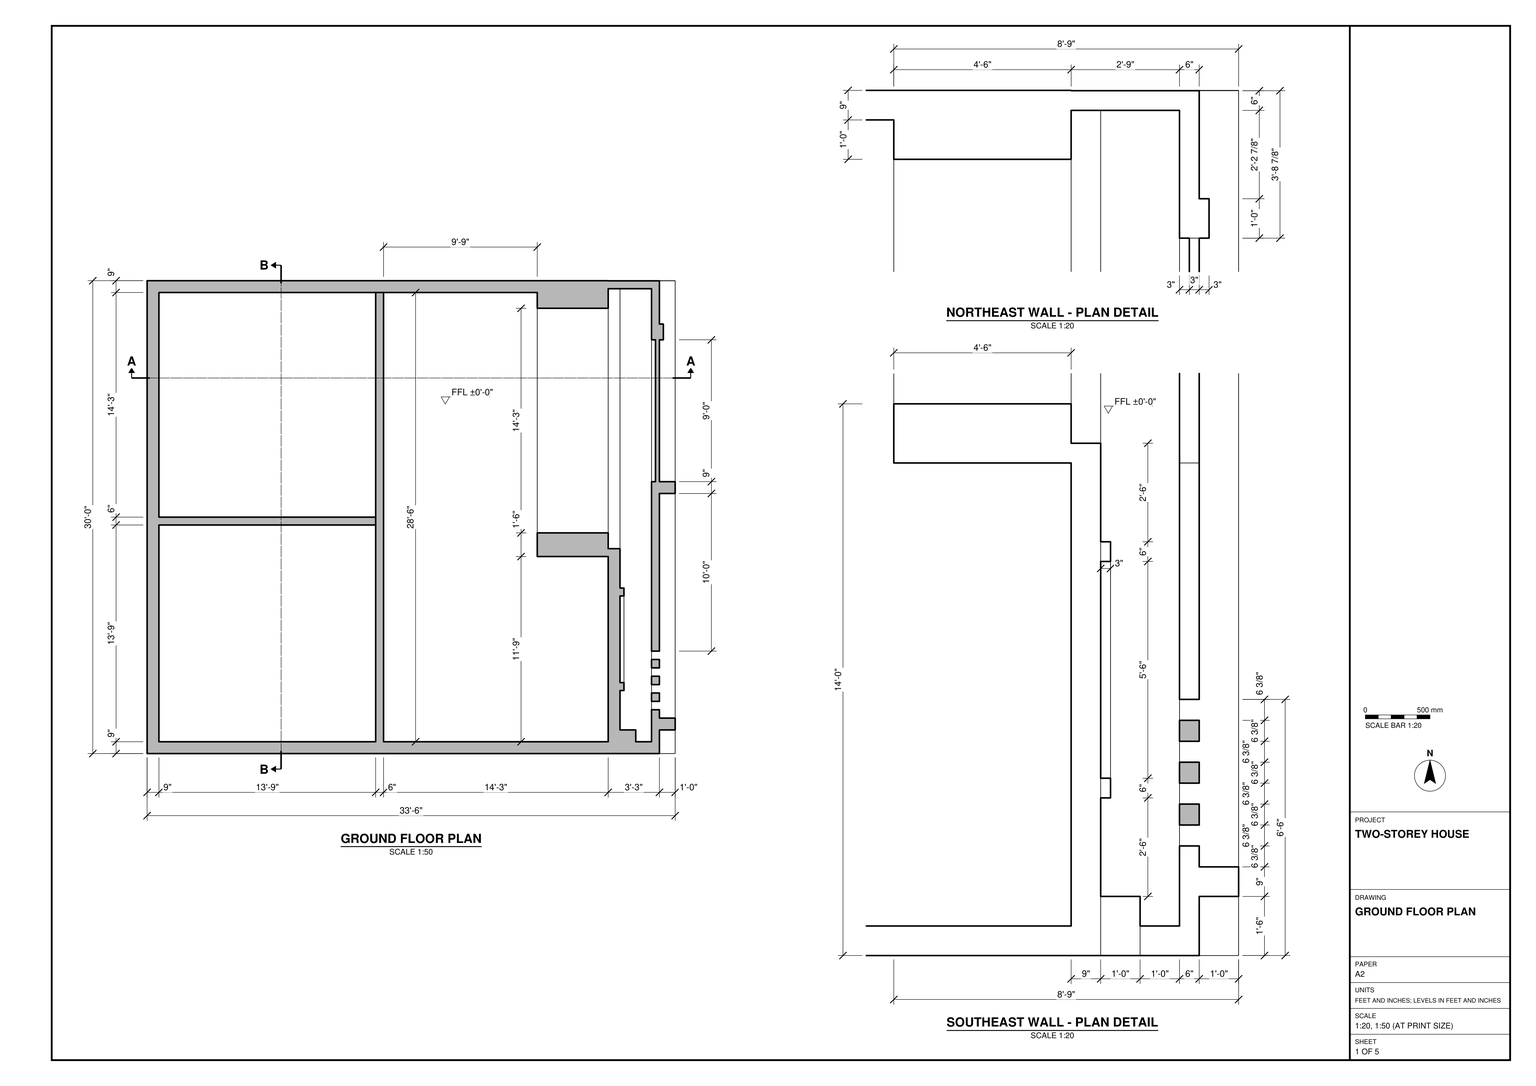
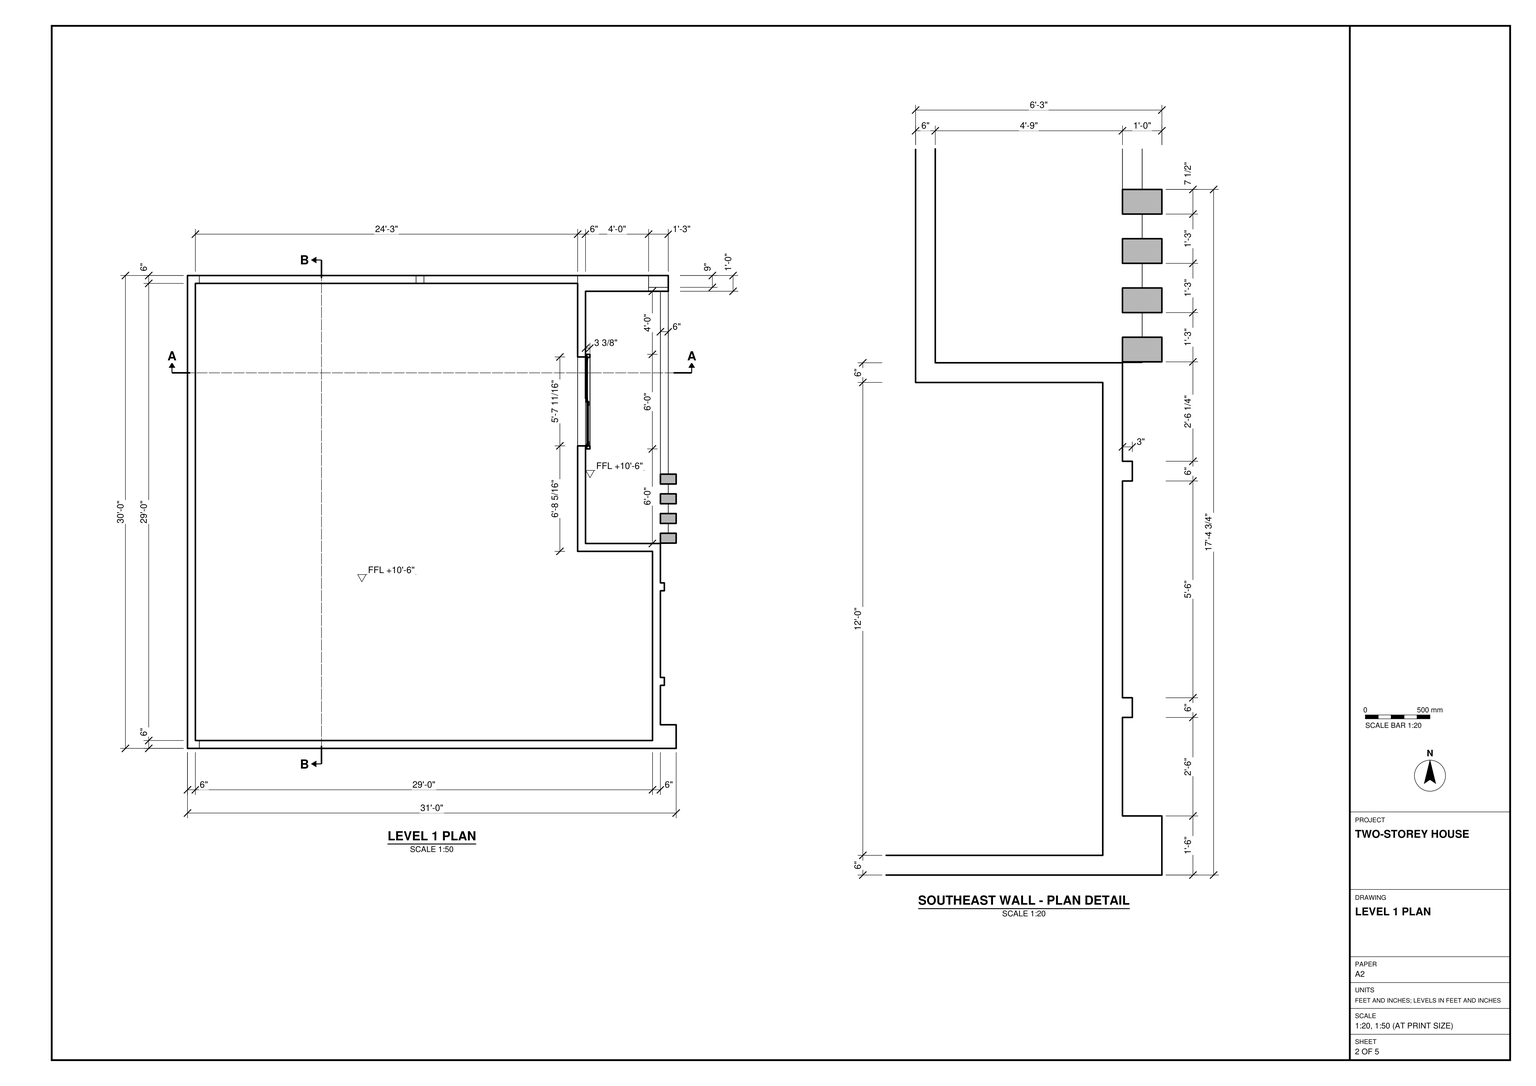
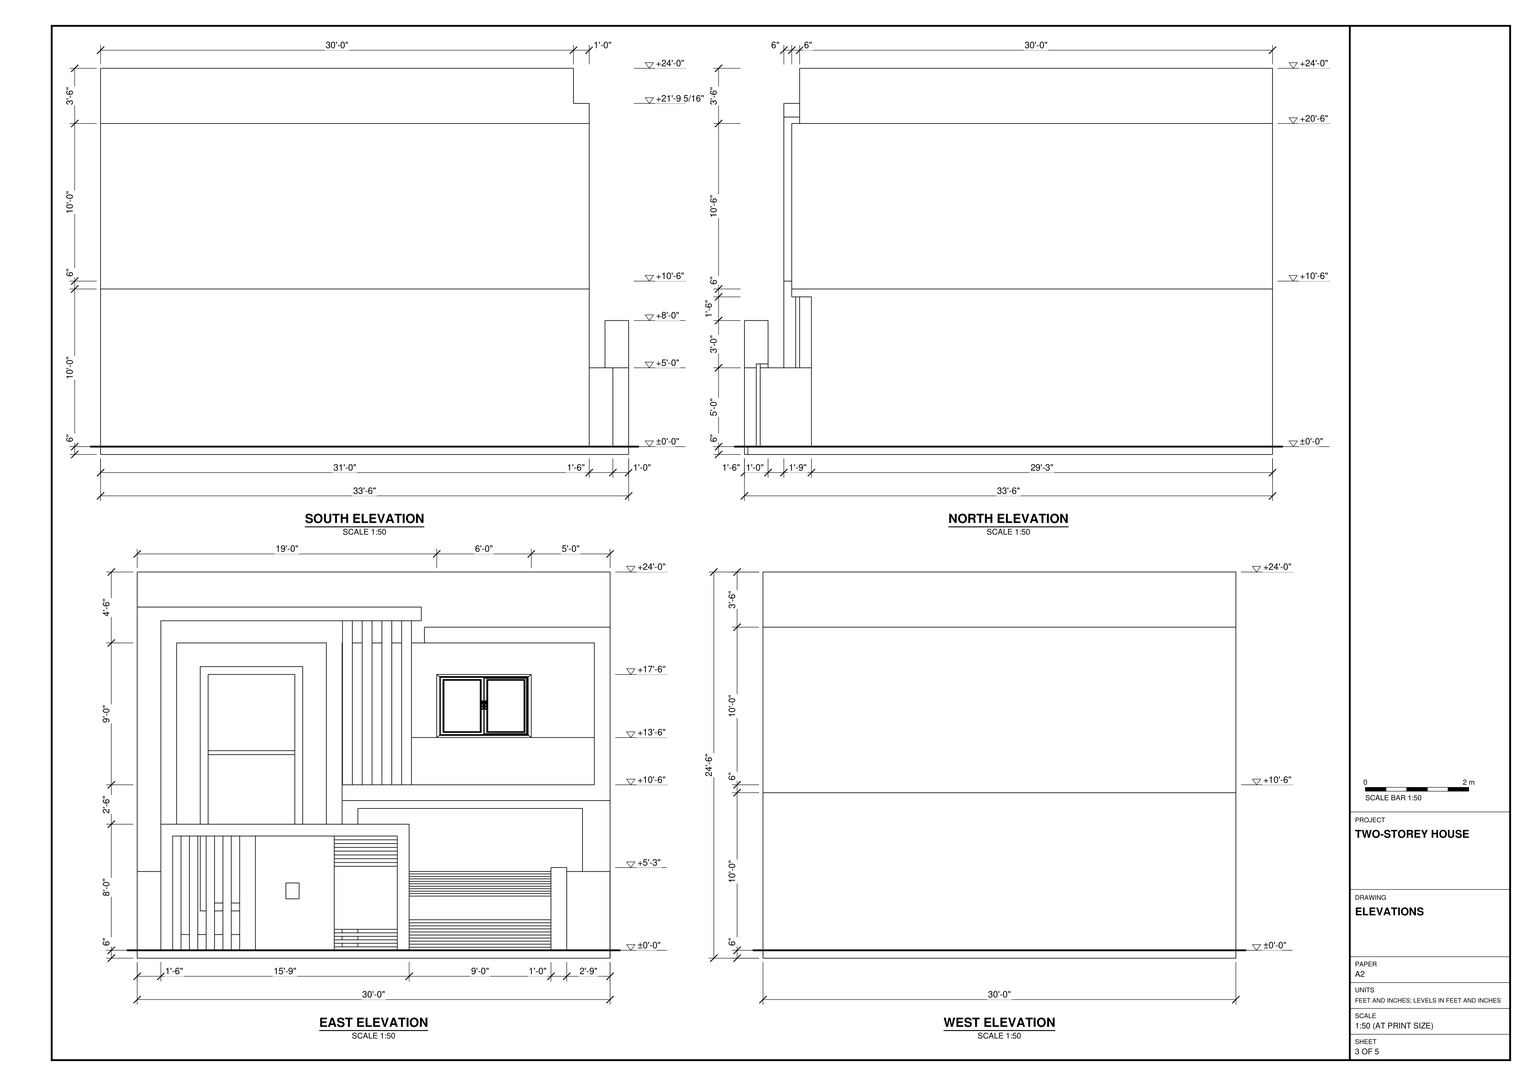
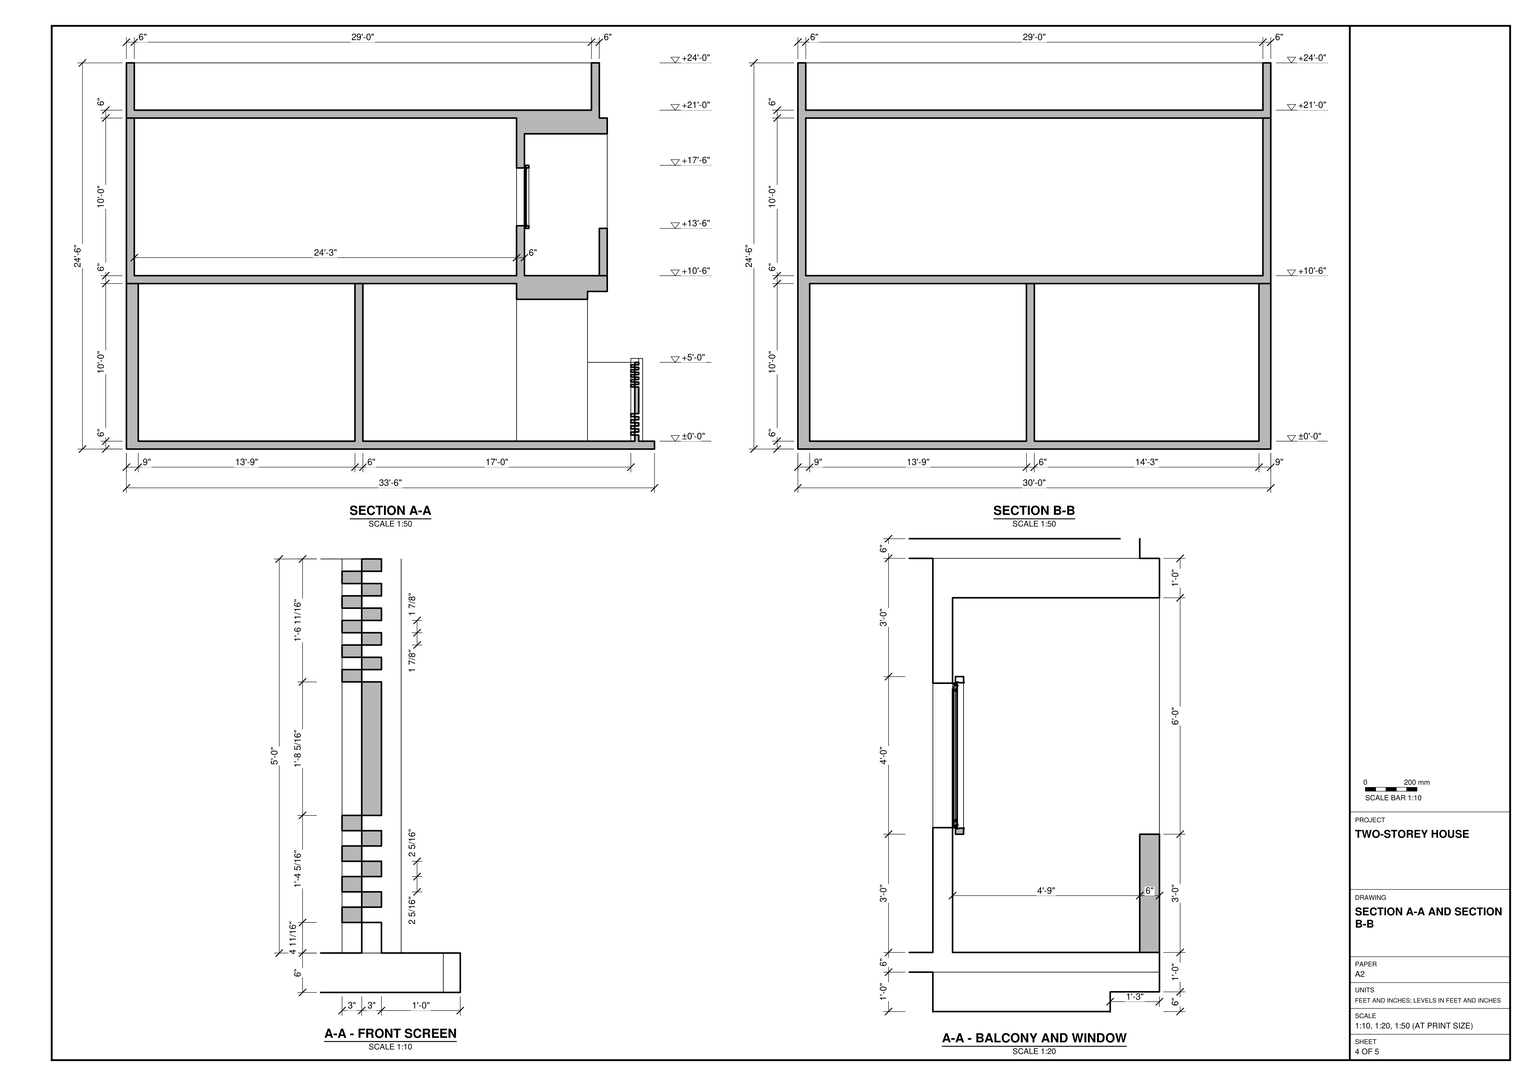
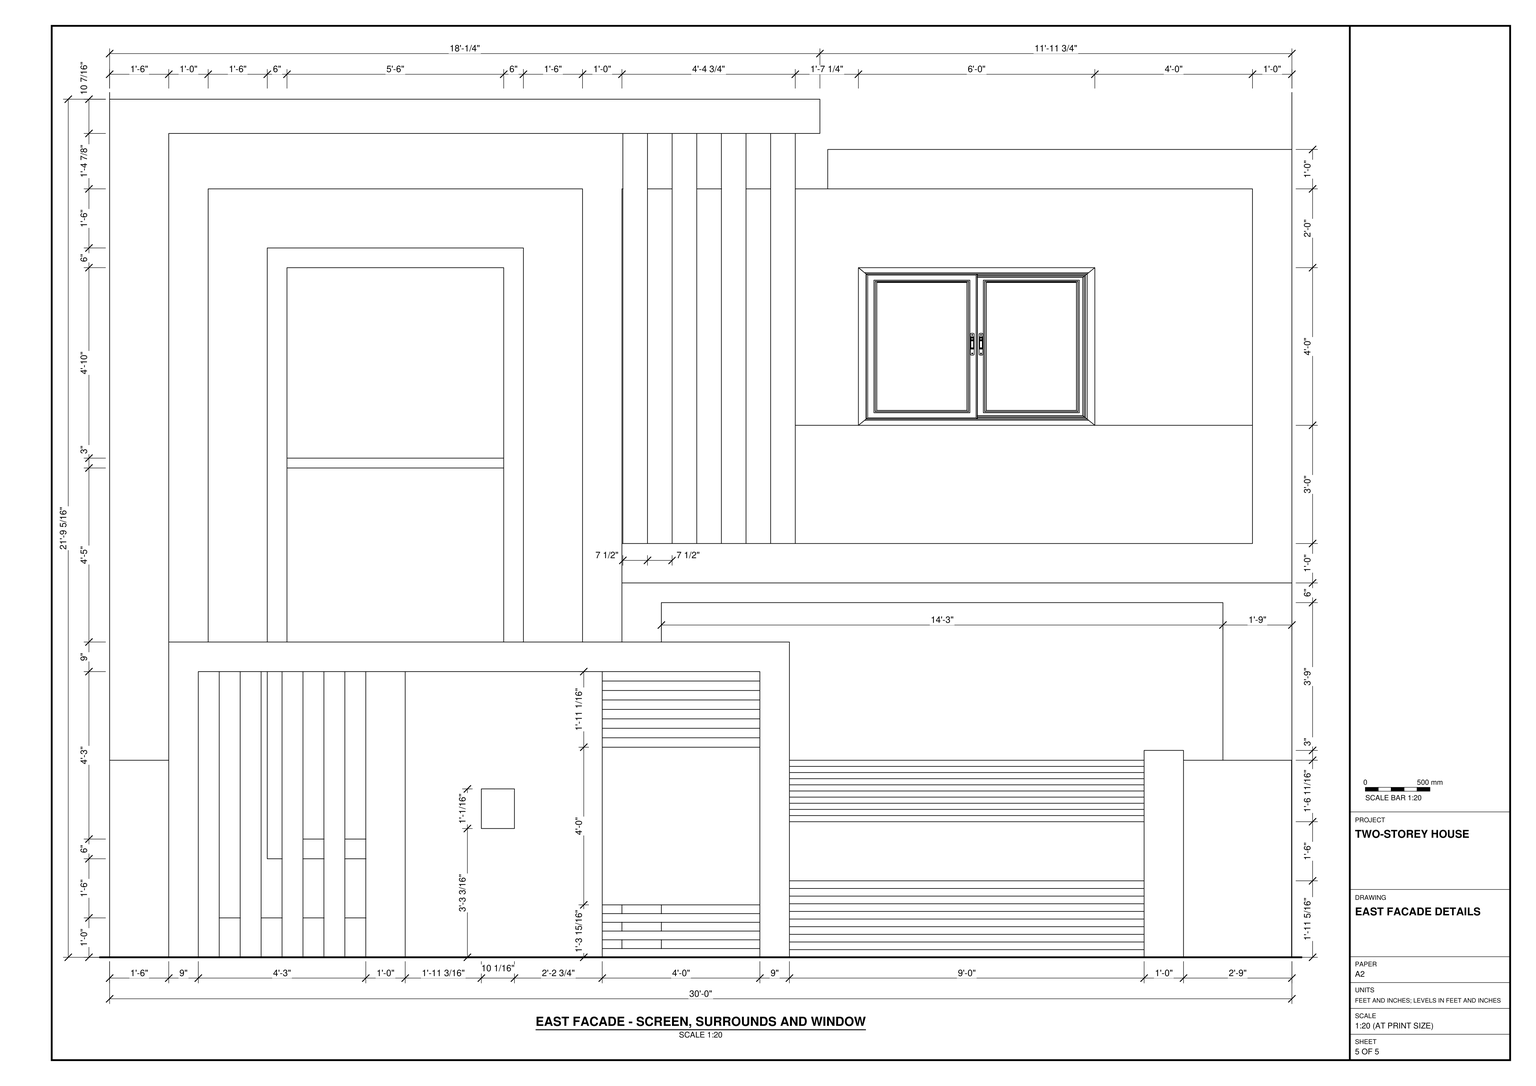
Build the two-storey house in SketchUp from task_files/diagram_01.pdf. Work in feet and inches. Orient the model with east–west along the x-axis and north–south along the y-axis. The overall extents, including the projecting east frontage and the base slab, are 33'-6" by 30'-0" by 24'-6". Set the ground finished floor at ±0'-0" and the upper finished floor at +10'-6". The parapet top is at +24'-0"; the overall height includes the 6" slab below the ground floor datum.

Follow the plans for wall positions and thicknesses. On the ground floor, use the north–south partition and its westward return to define the two western rooms. Use the enlarged east wall details to model the recesses and projections rather than treating the frontage as a single flat wall. Form the upper floor slab, the stepped upper perimeter, the flat roof and its parapet. Match the east elevation’s projecting frames, vertical fins, recessed window and lower frontage screen, keeping the solid panels distinct from the slatted sections.

Keep walls, slabs and roof as separate groups or components. Keep any furniture or joinery shown as separate pieces and use components for repeated parts such as matching fins. Any decor or loose items shown may be represented by suitable library components. Save one SketchUp model as output_files/two_storey_house_with_a_screened_east_facade.skp.

# SketchUp Ruby script. Lengths in inches.
U = 1.inch
M = Sketchup.active_model
def pt(a) = Geom::Point3d.new(a.map { |v| v * U })
def face(e, loops, mat)
  f = e.add_face(loops[0].map { |a| pt(a) })
  loops[1..].each { |l| e.add_face(l.map { |a| pt(a) }).erase! }
  f.material = f.back_material = mat if mat
  f
end
# faces: each face lists its corners as indices into pts; further lists are holes
def faces(e, pts, list, mat = nil) = list.each { |f| face(e, (f[0].is_a?(Array) ? f : [f]).map { |l| l.map { |i| pts[i] } }, mat) }
# xy, xz, yz: faces in a plane at the given z, y or x. An outline is a flat list of corners, or four numbers for a rectangle; further outlines are holes
def ring(l) = l.size == 4 ? [[l[0], l[1]], [l[2], l[1]], [l[2], l[3]], [l[0], l[3]]] : l.each_slice(2).to_a
def flat(e, list, mat, &to3) = list.each { |f| face(e, (f[0].is_a?(Array) ? f : [f]).map { |l| ring(l).map { |u, v| to3.(u, v) } }, mat) }
def xy(e, z, list, mat = nil) = flat(e, list, mat) { |x, y| [x, y, z] }
def xz(e, y, list, mat = nil) = flat(e, list, mat) { |x, z| [x, y, z] }
def yz(e, x, list, mat = nil) = flat(e, list, mat) { |y, z| [x, y, z] }
def lines(e, pts, list) = list.each { |a, b| e.add_line(pt(pts[a]), pt(pts[b])) }
# prism: a flat outline (further loops are holes) pulled along v
def prism(e, loops, v, mat = nil)
  f = face(e, loops, mat); d = Geom::Vector3d.new(v.map { |x| x * U })
  f.pushpull(f.normal.samedirection?(d) ? d.length : -d.length)
end
def box(e, o, s, mat = nil) = prism(e, [[o, [o[0] + s[0], o[1], o[2]], [o[0] + s[0], o[1] + s[1], o[2]], [o[0], o[1] + s[1], o[2]]]], [0, 0, s[2]], mat)
def at(x, y, z, deg = 0) = Geom::Transformation.translation(pt([x, y, z])) * Geom::Transformation.rotation(ORIGIN, Z_AXIS, deg.degrees)
def axes(o, x, y, z) = Geom::Transformation.new([*x, 0, *y, 0, *z, 0, *pt(o).to_a, 1])
def part(name) = M.definitions.add(name)
# library, detail: a bought-in or finely detailed component or shape, given as its bounding box
def library(name, o, s) = part(name).tap { |d| box(d.entities, o, s) }
def detail(e, o, s) = box(e.add_group.entities, o, s)
def put(e, d, t, mat = nil) = e.add_instance(d, t).tap { |i| i.material = mat if mat }
def group(e, t, mat = nil) = e.add_group.tap { |g| g.transformation = t; g.material = mat if mat }.entities
root = M.entities
M.materials.add("Carpet_04_1K").color = [43, 65, 85]
M.materials.add("Glass_Basic_01").color = [161, 173, 186]
M.materials["Glass_Basic_01"].alpha = 0.25
M.materials.add("H01_Misty_Ice").color = [204, 255, 255]
M.materials.add("I01_Sky_Frost").color = [241, 228, 255]
M.materials.add("J07_Grape_Bloom").color = [73, 0, 153]
M.materials.add("M01_Silver_Fog").color = [224, 224, 224]
M.materials.add("Wood_Veneer_15_1K").color = [103, 69, 45]
c1 = library("mesh-166",[-1553.69,-2604.3125,-42.18],[1702.88,1401.6,88.28])
p = [[354,150,258],[360,150,258]]
lines(root,p,[[0,1]])
g1 = group(root,at(304.52,281.23,221.76))
put(g1,c1,axes([0.14,12.46,29.44],[0,0.04228,0],[0,0,0.03425],[0.03937,0,0]))
g2 = group(root,at(0,0,-6),"I01_Sky_Frost")
xy(g2,0,[[0,0,0,360,402,359.91,402,0],[402,359.91,0,360,402,360]])
xy(g2,6,[[360,0,372,18],[390,0,402,18],[9,9,174,174],[180,9,351,9,351,150,297,150,297,351,180,351],[372,9,384,9,384,207,387,207,387,315,384,315,384,353.9,360,353.9,360,18,372,18],
  [390,27,402,27,402,198,390,198,390,78,384,78,384,71.625,390,71.625,390,65.25,384,65.25,384,58.875,390,58.875,390,52.5,384,52.5,384,46.125,390,46.125,390,39.75,384,39.75,384,33.375,390,33.375],[351,156,360,353.9],[297,168,351,339],[9,180,174,351],[390,207,402,207,402,359.9,390,359.9,390,327,393,327,393,315,390,315],
  [399.42,359.9,402,359.9,351,359.93,0,360],[351,359.9,360,359.93],[402,359.9,360,359.93,351,359.93],[360,359.9,372,359.9,367.03,359.92,360,359.93],[402,359.9,367.03,359.92,360,359.93],
  [367.03,359.92,360,359.96,360,359.93],[351,359.93,351,360,0,360],[351,359.93,360,359.93,360,359.96,351,360],[360,359.96,360,360,351,360]])
xy(g2,8.66,[[384,150,390,198]])
xy(g2,10.66,[[384,207,390,315]])
xy(g2,11.32,[[384,150,390,198]])
xy(g2,12.98,[[384,207,390,315]])
xy(g2,13.98,[[384,150,390,198]])
xy(g2,15.3125,[[384,207,390,315]])
xy(g2,16.65,[[384,150,390,198]])
xy(g2,17.64,[[384,207,390,315]])
xy(g2,19.31,[[384,150,390,198]])
xy(g2,19.97,[[384,207,390,315]])
xy(g2,21.97,[[384,150,390,198]])
xy(g2,22.3,[[384,207,390,315]])
xy(g2,24.625,[[384,207,390,315]])
xy(g2,26.95,[[384,207,390,315]])
xy(g2,36,[[360,48,363,126]])
xy(g2,42,[[360,54,363,120]])
xy(g2,47.28,[[384,207,390,315]])
xy(g2,49.15,[[384,207,390,315]])
xy(g2,51.03,[[384,207,390,315]])
xy(g2,52.9,[[384,207,390,315]])
xy(g2,54.77,[[384,207,390,315]])
xy(g2,56.64,[[384,207,390,315]])
xy(g2,58.51,[[384,207,390,315]])
xy(g2,60.38,[[384,207,390,315]])
xy(g2,62.26,[[384,207,390,315]])
xy(g2,64.13,[[384,207,390,315]])
xy(g2,66,[[372,0,390,0,390,18,384,18,384,9,372,9],[387,207,390,315],[384,327,390,327,390,359.9,351,359.9,351,353.9,384,353.9]])
xy(g2,69,[[384,315,393,327]])
xy(g2,69.97,[[384,150,390,198]])
xy(g2,72.85,[[384,150,390,198]])
xy(g2,75.73,[[384,150,390,198]])
xy(g2,78.61,[[384,150,390,198]])
xy(g2,81.48,[[384,150,390,198]])
xy(g2,84.36,[[384,150,390,198]])
xy(g2,87.24,[[384,150,390,198]])
xy(g2,90.12,[[384,150,390,198]])
xy(g2,93,[[390,27,390,33.375,384,33.375,384,39.75,390,39.75,390,46.125,384,46.125,384,52.5,390,52.5,390,58.875,384,58.875,384,65.25,390,65.25,390,71.625,384,71.625,384,78,390,78,390,198,402,198,402,27]],"Wood_Veneer_15_1K")
xy(g2,102,[[384,18,402,207]])
xy(g2,114,[[297,168,351,339]])
xy(g2,120,[[351,156,366,351],[351,351,366,360]])
xy(g2,126,[[0,0,9,360],[9,9,174,174],[174,9,180,351],[180,9,180,351,297,351,297,150,351,150,351,9],[9,174,174,180],
  [9,180,174,351],[9,351,174,360],[174,351,180,360],[180,351,297,360]])
xy(g2,132,[[6,6,354,6,354,150,297,150,297,354,6,354],[303,156,366,156,366,156.28,360,156.28,360,163.78,366,163.78,366,171.28,360,171.28,360,178.78,366,178.78,366,186.28,360,186.28,360,193.78,366,193.78,366,201.28,360,201.28,360,348,303,348],[360,156.28,366,163.78],[366,156.28,372,163.78],[360,171.28,366,178.78],
  [366,171.28,372,178.78],[360,186.28,366,193.78],[366,186.28,372,193.78],[360,201.28,366,348],[366,201.28,372,208.78]])
xy(g2,168,[[360,208.78,366,348]])
xy(g2,170,[[297,230,303,298]])
xy(g2,214,[[297,230,303,298]])
xy(g2,216,[[360,54,363,120]])
xy(g2,222,[[360,48,363,126]])
xy(g2,240,[[303,156,303,348,366,348,366,218.66,360,218.66,360,156]])
xy(g2,252,[[0,0,6,354],[6,6,6,354,297,354,297,150,354,150,354,6],[360,218.66,366,360],[0,354,303,360]])
xy(g2,256.875,[[360,18,372,156.28],[360,163.78,372,171.28],[360,178.78,372,186.28],[360,193.78,372,201.28],[360,208.78,372,216.28]],"Wood_Veneer_15_1K")
xy(g2,258,[[6,6,354,354]])
xy(g2,267.3,[[360,0,372,216.28]],"Wood_Veneer_15_1K")
xy(g2,294,[[[0,0,360,360],[6,6,354,354]]])
xz(g2,0,[[0,0,402,6],[0,6,372,126],[372,6,390,66],[0,126,372,252],[0,252,372,252,372,267.3,360,267.3,360,294,0,294]])
xz(g2,6,[[6,132,354,252],[6,258,354,294]])
xz(g2,9,[[9,6,174,126],[180,6,351,126],[372,6,384,66]])
xz(g2,18,[[390,6,402,66],[384,66,402,102]])
xz(g2,18,[[360,6,372,256.875]],"Wood_Veneer_15_1K")
xz(g2,27,[[390,6,402,66],[390,66,402,93]],"Wood_Veneer_15_1K")
xz(g2,33.375,[[384,6,390,93]])
xz(g2,39.75,[[384,6,390,93]])
xz(g2,46.125,[[384,6,390,93]])
xz(g2,48,[[360,36,363,222]])
xz(g2,52.5,[[384,6,390,93]])
xz(g2,54,[[360,42,363,97],[360,97,363,100],[360,100,363,155],[360,155,363,158],[360,158,363,216]])
xz(g2,58.875,[[384,6,390,93]])
xz(g2,65.25,[[384,6,390,93]])
xz(g2,71.625,[[384,6,390,93]])
xz(g2,78,[[384,6,390,93]])
xz(g2,120,[[360,42,363,97],[360,97,363,100],[360,100,363,120],[360,120,363,126],[360,126,363,132],
  [360,132,363,155],[360,155,363,158],[360,158,363,216]])
xz(g2,126,[[360,36,363,120],[360,120,363,126],[360,126,363,132],[360,132,363,222]])
xz(g2,150,[[297,6,303,126],[303,6,351,126],[384,8.66,390,11.32],[384,13.98,390,16.65],[384,19.31,390,21.97],
  [384,69.97,390,72.85],[384,75.73,390,78.61],[384,81.48,390,84.36],[384,87.24,390,90.12],[297,132,354,252]])
xz(g2,156,[[351,6,360,120],[360,120,366,126],[360,126,366,132],[303,132,360,240]])
xz(g2,156.28,[[360,132,372,256.875]])
xz(g2,163.78,[[360,132,372,256.875]])
xz(g2,168,[[297,6,351,114]])
xz(g2,171.28,[[360,132,372,256.875]])
xz(g2,174,[[9,6,174,126]])
xz(g2,178.78,[[360,132,372,256.875]])
xz(g2,180,[[9,6,174,126]])
xz(g2,186.28,[[360,132,372,256.875]])
xz(g2,193.78,[[360,132,372,256.875]])
xz(g2,198,[[390,6,402,6,402,93,390,93,390,90.12,384,90.12,384,87.24,390,87.24,390,84.36,384,84.36,384,81.48,390,81.48,390,78.61,384,78.61,384,75.73,390,75.73,390,72.85,384,72.85,384,69.97,390,69.97,390,21.97,384,21.97,384,19.31,390,19.31,390,16.65,384,16.65,384,13.98,390,13.98,390,11.32,384,11.32,384,8.66,390,8.66]],"Wood_Veneer_15_1K")
xz(g2,201.28,[[360,132,372,256.875]])
xz(g2,207,[[384,6,387,10.66],[390,6,390,10.66,387,10.66,387,12.98,390,12.98,390,15.3125,387,15.3125,387,17.64,390,17.64,390,19.97,387,19.97,387,22.3,390,22.3,390,24.625,387,24.625,387,26.95,390,26.95,390,47.28,387,47.28,387,49.15,390,49.15,390,51.03,387,51.03,387,52.9,390,52.9,390,54.77,387,54.77,387,56.64,390,56.64,390,58.51,387,58.51,387,60.38,390,60.38,390,62.26,387,62.26,387,64.13,390,64.13,390,66,402,66,402,6],[384,10.66,387,12.98],[384,12.98,387,15.3125],[384,15.3125,387,17.64],
  [384,17.64,387,19.97],[384,19.97,387,22.3],[384,22.3,387,24.625],[384,24.625,387,26.95],[384,26.95,387,47.28],
  [384,47.28,387,49.15],[384,49.15,387,51.03],[384,51.03,387,52.9],[384,52.9,387,54.77],[384,54.77,387,56.64],
  [384,56.64,387,58.51],[384,58.51,387,60.38],[384,60.38,387,62.26],[384,62.26,387,64.13],[384,64.13,387,66],
  [384,66,402,102]])
xz(g2,208.78,[[366,132,366,168,360,168,360,256.875,372,256.875,372,132]])
xz(g2,216.28,[[360,256.875,372,267.3]],"Wood_Veneer_15_1K")
xz(g2,218.66,[[360,240,366,252]])
xz(g2,230,[[297,170,303,214]])
xz(g2,298,[[297,170,303,214]])
xz(g2,315,[[384,6,387,10.66],[390,6,393,6,393,69,390,69,390,64.13,387,64.13,387,62.26,390,62.26,390,60.38,387,60.38,387,58.51,390,58.51,390,56.64,387,56.64,387,54.77,390,54.77,390,52.9,387,52.9,387,51.03,390,51.03,390,49.15,387,49.15,387,47.28,390,47.28,390,26.95,387,26.95,387,24.625,390,24.625,390,22.3,387,22.3,387,19.97,390,19.97,390,17.64,387,17.64,387,15.3125,390,15.3125,390,12.98,387,12.98,387,10.66,390,10.66],[384,10.66,387,12.98],[384,12.98,387,15.3125],[384,15.3125,387,17.64],
  [384,17.64,387,19.97],[384,19.97,387,22.3],[384,22.3,387,24.625],[384,24.625,387,26.95],[384,26.95,387,47.28],
  [384,47.28,387,49.15],[384,49.15,387,51.03],[384,51.03,387,52.9],[384,52.9,387,54.77],[384,54.77,387,56.64],
  [384,56.64,387,58.51],[384,58.51,387,60.38],[384,60.38,387,62.26],[384,62.26,387,64.13],[384,64.13,387,66],
  [384,66,390,69]])
xz(g2,327,[[390,6,393,69],[384,66,390,69]])
xz(g2,339,[[297,6,351,114]])
xz(g2,348,[[303,132,360,132,360,168,366,168,366,240,303,240]])
xz(g2,351,[[9,6,174,126],[174,6,180,126],[180,6,297,126]])
xz(g2,353.9,[[351,6,384,66]])
xz(g2,354,[[6,132,297,252],[6,258,354,294]])
xz(g2,359.9,[[399.42,5.96,399.42,6,402,6],[351,6,390,66]])
xz(g2,360,[[0,6,0,126,366,126,366,120,351,120,351,6],[0,126,366,252],[0,252,360,294]])
yz(g2,0,[[0,0,360,6],[0,6,360,126],[0,126,360,252],[0,252,360,294]])
yz(g2,6,[[6,132,354,252],[6,258,354,294]])
yz(g2,9,[[9,6,174,126],[180,6,351,126]])
yz(g2,174,[[9,6,174,126],[174,6,180,126],[180,6,351,126]])
yz(g2,180,[[9,6,351,126]])
yz(g2,297,[[150,6,150,126,351,126,351,6,339,6,339,114,168,114,168,6],[[150,132,354,252],[230,170,298,214]]])
yz(g2,303,[[[228,168,300,216],[230,170,298,214]]])
yz(g2,303,[[[156,132,348,240],[228,168,300,216]]],"I01_Sky_Frost")
yz(g2,351,[[9,6,150,126]])
yz(g2,351,[[156,6,168,6,168,114,339,114,339,6,353.9,6,353.9,66,359.9,66,359.9,6,360,6,360,120,156,120]],"Carpet_04_1K")
yz(g2,354,[[6,132,150,252],[6,258,156,294],[156,258,354,294]])
yz(g2,360,[[156.28,132,163.78,240],[171.28,132,178.78,240],[186.28,132,193.78,240],[163.78,240,171.28,256.875],[178.78,240,186.28,256.875],
  [193.78,240,201.28,256.875]])
yz(g2,360,[[[18,6,156,6,156,240,156.28,240,156.28,256.875,18,256.875],[30,18,144,240]],[[30,18,144,240],[48,36,126,222]],[208.78,240,218.66,240,218.66,252,360,252,360,294,0,294,0,267.3,216.28,267.3,216.28,256.875,208.78,256.875]],"Carpet_04_1K")
yz(g2,360,[[201.28,132,201.28,240,208.78,240,208.78,168,348,168,348,132]],"Glass_Basic_01")
yz(g2,360,[[54,100,120,155],[54,158,120,216]],"H01_Misty_Ice")
yz(g2,360,[[54,42,120,97]],"I01_Sky_Frost")
yz(g2,360,[[54,97,120,100],[54,155,120,158]],"J07_Grape_Bloom")
yz(g2,363,[[[48,36,126,222],[54,42,120,216]]])
yz(g2,366,[[208.78,132,348,168]],"Glass_Basic_01")
yz(g2,366,[[156,120,360,120,360,252,218.66,252,218.66,240,348,240,348,132,156,132]],"M01_Silver_Fog")
yz(g2,372,[[156.28,132,163.78,256.875],[171.28,132,178.78,256.875],[186.28,132,193.78,256.875],[201.28,132,208.78,256.875]],"Carpet_04_1K")
yz(g2,372,[[9,6,18,6,18,256.875,216.28,256.875,216.28,267.3,0,267.3,0,66,9,66]],"Wood_Veneer_15_1K")
yz(g2,384,[[9,6,18,66],[[18,6,18,102,207,102,207,66,198,66,198,90.12,150,90.12,150,87.24,198,87.24,198,84.36,150,84.36,150,81.48,198,81.48,198,78.61,150,78.61,150,75.73,198,75.73,198,72.85,150,72.85,150,69.97,198,69.97,198,66,207,66,207,6,78,6,78,93,71.625,93,71.625,6,65.25,6,65.25,93,58.875,93,58.875,6,52.5,6,52.5,93,46.125,93,46.125,6,39.75,6,39.75,93,33.375,93,33.375,6],[150,19.31,198,21.97],[150,13.98,198,16.65],[150,8.66,198,11.32]],[315,6,315,69,327,69,327,66,353.9,66,353.9,6],[207,10.66,315,12.98],[207,15.3125,315,17.64],
  [207,19.97,315,22.3],[207,24.625,315,26.95],[207,47.28,315,49.15],[207,51.03,315,52.9],[207,54.77,315,56.64],
  [207,58.51,315,60.38],[207,62.26,315,64.13],[150,69.97,198,72.85],[150,75.73,198,78.61],[150,81.48,198,84.36],
  [150,87.24,198,90.12]])
yz(g2,387,[[207,6,315,66]])
yz(g2,390,[[0,6,18,66],[27,6,33.375,93],[39.75,6,46.125,93],[52.5,6,58.875,93],[65.25,6,71.625,93],
  [78,6,90,93],[150,6,198,8.66],[207,6,315,8.33],[207,8.33,315,10.66],[150,11.32,198,13.98],
  [207,12.98,315,15.3125],[150,16.65,198,19.31],[207,17.64,315,19.97],[207,22.3,315,24.625],[207,26.95,315,29.28],
  [207,49.15,315,51.03],[207,52.9,315,54.77],[207,56.64,315,58.51],[207,60.38,315,62.26],[207,64.13,315,66],
  [150,72.85,198,75.73],[150,78.61,198,81.48],[150,84.36,198,87.24],[150,90.12,198,93]])
yz(g2,390,[[113.19,45.21,123.26,57.28]],"H01_Misty_Ice")
yz(g2,390,[[327,6,359.9,66],[150,21.97,198,69.97],[207,29.28,315,47.28]],"I01_Sky_Frost")
yz(g2,390,[[[90,6,150,93],[113.19,45.21,123.26,57.28]]],"Wood_Veneer_15_1K")
yz(g2,393,[[315,6,327,69]])
yz(g2,402,[[0,0,359.9,6],[359.9,0,359.91,0,359.9,6],[359.91,0,359.9,6,360,0]])
yz(g2,402,[[18,6,27,6,27,93,198,93,198,6,207,6,207,102,18,102]],"I01_Sky_Frost")
p = [[402,359.91,0],[0,360,0],[399.42,359.9,5.96],[402,359.9,6],[0,360,6],[399.42,359.9,6],
  [399.42,360,0],[402,360,0],[384,198,93],[384,198,90.12],[480.87,360,0],[480.87,359.9,0],
  [354,150,252],[360,150,252],[354,6,252],[360,6,252]]
faces(g2,p,[[0,1,2,3],[4,5,2,1],[6,2,1],[7,3,2,6]])
lines(g2,p,[[8,9],[10,11],[12,13],[14,15]])
